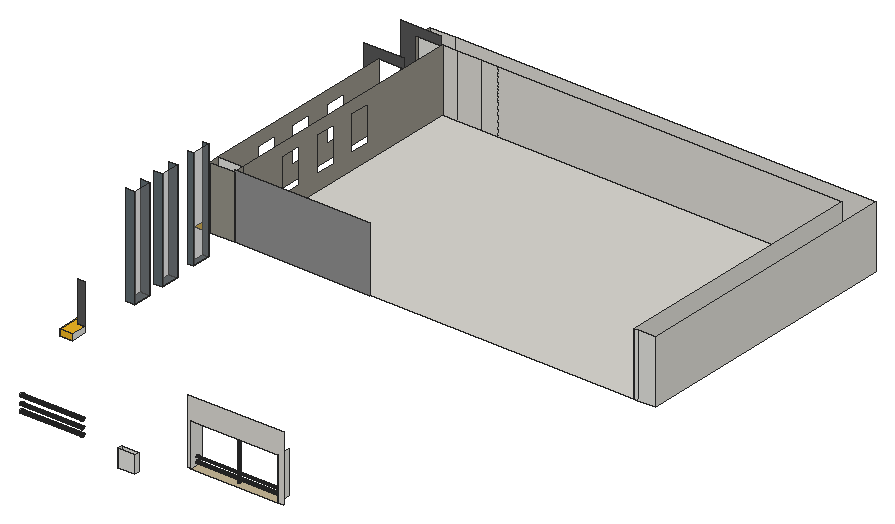
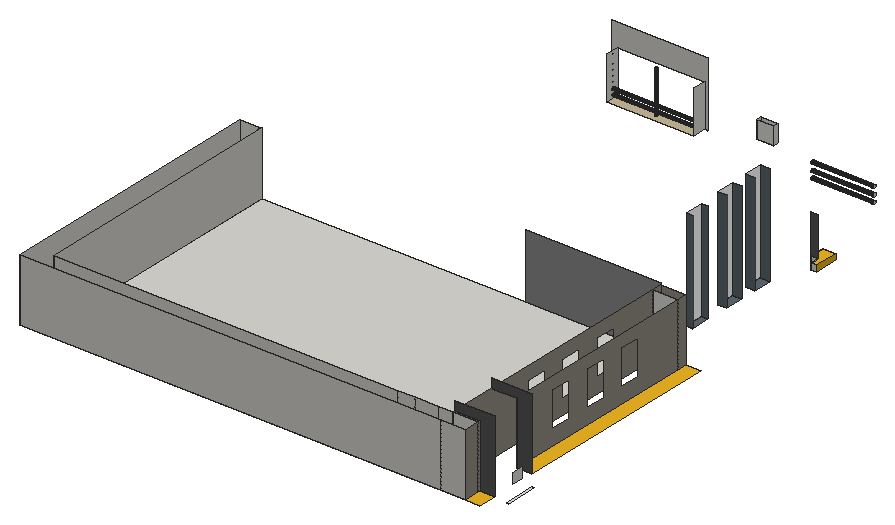
# SketchUp Ruby script. Lengths in inches.
U = 1.inch
M = Sketchup.active_model
def pt(a) = Geom::Point3d.new(a.map { |v| v * U })
def face(e, loops, mat)
  f = e.add_face(loops[0].map { |a| pt(a) })
  loops[1..].each { |l| e.add_face(l.map { |a| pt(a) }).erase! }
  f.material = f.back_material = mat if mat
  f
end
# faces: each face lists its corners as indices into pts; further lists are holes
def faces(e, pts, list, mat = nil) = list.each { |f| face(e, (f[0].is_a?(Array) ? f : [f]).map { |l| l.map { |i| pts[i] } }, mat) }
# xy, xz, yz: faces in a plane at the given z, y or x. An outline is a flat list of corners, or four numbers for a rectangle; further outlines are holes
def ring(l) = l.size == 4 ? [[l[0], l[1]], [l[2], l[1]], [l[2], l[3]], [l[0], l[3]]] : l.each_slice(2).to_a
def flat(e, list, mat, &to3) = list.each { |f| face(e, (f[0].is_a?(Array) ? f : [f]).map { |l| ring(l).map { |u, v| to3.(u, v) } }, mat) }
def xy(e, z, list, mat = nil) = flat(e, list, mat) { |x, y| [x, y, z] }
def xz(e, y, list, mat = nil) = flat(e, list, mat) { |x, z| [x, y, z] }
def yz(e, x, list, mat = nil) = flat(e, list, mat) { |y, z| [x, y, z] }
def lines(e, pts, list) = list.each { |a, b| e.add_line(pt(pts[a]), pt(pts[b])) }
# prism: a flat outline (further loops are holes) pulled along v
def prism(e, loops, v, mat = nil)
  f = face(e, loops, mat); d = Geom::Vector3d.new(v.map { |x| x * U })
  f.pushpull(f.normal.samedirection?(d) ? d.length : -d.length)
end
def box(e, o, s, mat = nil) = prism(e, [[o, [o[0] + s[0], o[1], o[2]], [o[0] + s[0], o[1] + s[1], o[2]], [o[0], o[1] + s[1], o[2]]]], [0, 0, s[2]], mat)
def at(x, y, z, deg = 0) = Geom::Transformation.translation(pt([x, y, z])) * Geom::Transformation.rotation(ORIGIN, Z_AXIS, deg.degrees)
def axes(o, x, y, z) = Geom::Transformation.new([*x, 0, *y, 0, *z, 0, *pt(o).to_a, 1])
def part(name) = M.definitions.add(name)
# library, detail: a bought-in or finely detailed component or shape, given as its bounding box
def library(name, o, s) = part(name).tap { |d| box(d.entities, o, s) }
def detail(e, o, s) = box(e.add_group.entities, o, s)
def put(e, d, t, mat = nil) = e.add_instance(d, t).tap { |i| i.material = mat if mat }
def group(e, t, mat = nil) = e.add_group.tap { |g| g.transformation = t; g.material = mat if mat }.entities
root = M.entities
M.materials.add("[0045_Goldenrod]").color = [239, 181, 35]
M.materials.add("[Color M04]").color = [142, 142, 142]
M.materials.add("[Color M06]").color = [86, 86, 86]
M.materials.add("[Color M07]").color = [58, 58, 58]
M.materials.add("[Formica Graystone]").color = [149, 146, 135]
M.materials.add("[Formica Speckled Grey]").color = [94, 105, 111]
M.materials.add("[Quartz Light Brown]").color = [199, 184, 152]
M.materials.add("[Terrazzo Tile Light]").color = [219, 217, 210]
M.materials.add("[Translucent Glass Gray]1").color = [128, 128, 128]
M.materials["[Translucent Glass Gray]1"].alpha = 0.5
xy(root,388.58,[[0,731.17,2.5625,767.73]])
xy(root,390.15,[[220.22,108.25,239.85,114.1875]])
xy(root,396.69,[[329.08,144.78,328.77,144.82,328.48,144.9375,328.24,145.125,328.05,145.37,327.93,145.66,327.89,145.96,327.93,146.27,328.05,146.56,328.24,146.8,328.48,146.99,328.77,147.11,329.08,147.15,329.38,147.11,329.67,146.99,329.91,146.8,330.1,146.56,330.22,146.27,330.26,145.96,330.22,145.66,330.1,145.37,329.91,145.125,329.67,144.9375,329.38,144.82]])
xy(root,396.69,[[[280.22,138.52,379.09,153.42],[329.08,144.78,328.77,144.82,328.48,144.9375,328.24,145.125,328.05,145.37,327.93,145.66,327.89,145.96,327.93,146.27,328.05,146.56,328.24,146.8,328.48,146.99,328.77,147.11,329.08,147.15,329.38,147.11,329.67,146.99,329.91,146.8,330.1,146.56,330.22,146.27,330.26,145.96,330.22,145.66,330.1,145.37,329.91,145.125,329.67,144.9375,329.38,144.82]]],"[Quartz Light Brown]")
xy(root,396.875,[[25.28,483.625,53.375,495.58],[509.21,483.625,509.21,779.875,25.28,779.875,25.28,797.6875,533.375,797.6875,533.375,483.625]])
xy(root,396.875,[[8.375,483.625,25.28,724.47],[8.375,777.2,25.28,797.6875]],"[0045_Goldenrod]")
xy(root,396.875,[[53.375,483.625,509.21,779.875]],"[Terrazzo Tile Light]")
xy(root,397.66,[[38.625,253.03,38.625,280.03,45.3125,280.03,45.3125,270.46,53.375,270.46,53.375,253.03]],"[0045_Goldenrod]")
xy(root,404.29,[[53.375,329.18,63.8125,350.43],[53.375,369.37,62.6875,390.62],[53.375,417,60.4375,438.25]],"[Formica Speckled Grey]")
xy(root,404.47,[[38.625,253.03,53.375,253.03,53.375,270.46,45.3125,270.46,45.3125,280.03,38.625,280.03]],"[0045_Goldenrod]")
xz(root,108.25,[[220.22,390.15,239.85,409.78]])
xz(root,114.1875,[[220.22,390.15,239.85,409.78]])
xz(root,138.52,[[276.16,396.69,280.22,396.69,280.22,445.19,379.09,445.19,379.09,396.69,385.17,396.69,385.17,471,276.16,471]],"[Terrazzo Tile Light]")
xz(root,253.03,[[38.625,397.66,53.375,404.47]],"[0045_Goldenrod]")
xz(root,270.46,[[45.3125,397.66,53.375,404.47]])
xz(root,270.46,[[45.3125,404.47,53.375,449.66]],"[Color M06]")
xz(root,280.03,[[38.625,397.66,45.3125,404.47]])
xz(root,329.18,[[53.375,404.29,63.8125,519.67]],"[Formica Speckled Grey]")
xz(root,350.43,[[53.375,404.29,63.8125,519.67]],"[Formica Speckled Grey]")
xz(root,369.37,[[53.375,404.29,62.6875,519.67]],"[Formica Speckled Grey]")
xz(root,390.62,[[53.375,404.29,62.6875,519.67]],"[Formica Speckled Grey]")
xz(root,417,[[53.375,404.29,60.4375,519.67]],"[Formica Speckled Grey]")
xz(root,438.25,[[53.375,404.29,60.4375,519.67]],"[Formica Speckled Grey]")
xz(root,483.625,[[509.21,396.875,513.45,468.5],[513.45,396.875,533.375,468.5]])
xz(root,483.625,[[53.375,396.875,208.03,471]],"[Color M04]")
xz(root,483.625,[[25.28,396.875,53.375,468.5]],"[Formica Graystone]")
xz(root,495.58,[[25.28,396.875,53.375,468.5]])
xz(root,724.47,[[8.375,396.875,25.28,396.875,25.28,468.5,53.375,468.5,53.375,479.1875,8.375,479.1875]],"[Color M06]")
xz(root,777.2,[[8.375,396.875,8.375,479.1875,53.375,479.1875,53.375,468.5,25.28,468.5,25.28,396.875]],"[Color M06]")
xz(root,779.875,[[25.28,396.875,53.375,468.5]])
xz(root,779.875,[[53.375,396.875,70.21,468.5],[70.21,396.875,97.02,468.5],[97.02,396.875,116.75,468.5],[116.75,396.875,509.21,468.5]],"[Terrazzo Tile Light]")
xz(root,797.6875,[[25.28,396.875,53.375,468.5],[53.375,396.875,533.375,468.5]],"[Terrazzo Tile Light]")
yz(root,2.5625,[[745.75,403.69,759.0625,415.44]])
yz(root,25.28,[[483.625,396.875,495.58,468.5],[[495.58,396.875,724.47,468.5],[649.81,414.79,673.99,454.59],[600.93,414.79,625.12,454.59],[551.74,414.79,575.93,454.59]],[777.2,396.875,779.875,468.5],[779.875,396.875,797.6875,468.5]],"[Formica Graystone]")
yz(root,38.625,[[253.03,397.66,280.03,404.47]],"[0045_Goldenrod]")
yz(root,45.3125,[[270.46,397.66,280.03,404.47]])
yz(root,53.375,[[253.03,397.66,270.46,404.47]])
yz(root,53.375,[[483.625,396.875,495.58,468.5],[[495.58,396.875,779.875,468.5],[649.81,414.79,673.99,454.59],[600.93,414.79,625.12,454.59],[551.74,414.79,575.93,454.59]]],"[Formica Graystone]")
yz(root,60.4375,[[417,404.29,438.25,519.67]],"[Translucent Glass Gray]1")
yz(root,62.6875,[[369.37,404.29,390.62,519.67]],"[Translucent Glass Gray]1")
yz(root,63.8125,[[329.18,404.29,350.43,519.67]],"[Translucent Glass Gray]1")
yz(root,87.31,[[136.99,387.18,136.55,387.24,136.14,387.41,135.79,387.67,135.52,388.02,135.36,388.43,135.3,388.87,135.36,389.3,135.52,389.71,135.79,390.06,136.14,390.33,136.55,390.5,136.99,390.55,137.42,390.5,137.83,390.33,138.18,390.06,138.45,389.71,138.62,389.3,138.67,388.87,138.62,388.43,138.45,388.02,138.18,387.67,137.83,387.41,137.42,387.24],[136.99,394.8,136.55,394.86,136.14,395.03,135.79,395.3,135.52,395.65,135.36,396.06,135.3,396.49,135.36,396.93,135.52,397.34,135.79,397.69,136.14,397.95,136.55,398.12,136.99,398.18,137.42,398.12,137.83,397.95,138.18,397.69,138.45,397.34,138.62,396.93,138.67,396.49,138.62,396.06,138.45,395.65,138.18,395.3,137.83,395.03,137.42,394.86],[136.99,403.55,136.55,403.61,136.14,403.78,135.79,404.05,135.52,404.4,135.36,404.81,135.3,405.24,135.36,405.68,135.52,406.09,135.79,406.44,136.14,406.7,136.55,406.87,136.99,406.93,137.42,406.87,137.83,406.7,138.18,406.44,138.45,406.09,138.62,405.68,138.67,405.24,138.62,404.81,138.45,404.4,138.18,404.05,137.83,403.78,137.42,403.61]])
yz(root,220.22,[[108.25,390.15,114.1875,409.78]])
yz(root,239.85,[[108.25,390.15,114.1875,409.78]])
yz(root,280.22,[[[138.52,396.69,153.42,445.19],[145.73,399.5,145.38,399.55,145.05,399.6875,144.76,399.91,144.54,400.19,144.41,400.52,144.36,400.88,144.41,401.23,144.54,401.57,144.76,401.85,145.05,402.07,145.38,402.21,145.73,402.25,146.09,402.21,146.42,402.07,146.71,401.85,146.92,401.57,147.0625,401.23,147.11,400.88,147.0625,400.52,146.92,400.19,146.71,399.91,146.42,399.6875,146.09,399.55],[145.73,434.63,145.38,434.67,145.05,434.8125,144.76,435.03,144.54,435.32,144.41,435.65,144.36,436,144.41,436.36,144.54,436.69,144.76,436.97,145.05,437.19,145.38,437.33,145.73,437.38,146.09,437.33,146.42,437.19,146.71,436.97,146.92,436.69,147.0625,436.36,147.11,436,147.0625,435.65,146.92,435.32,146.71,435.03,146.42,434.8125,146.09,434.67],[145.73,405.25,145.38,405.3,145.05,405.4375,144.76,405.66,144.54,405.94,144.41,406.27,144.36,406.63,144.41,406.98,144.54,407.32,144.76,407.6,145.05,407.82,145.38,407.96,145.73,408,146.09,407.96,146.42,407.82,146.71,407.6,146.92,407.32,147.0625,406.98,147.11,406.63,147.0625,406.27,146.92,405.94,146.71,405.66,146.42,405.4375,146.09,405.3],[145.73,429.69,145.38,429.74,145.05,429.875,144.76,430.09,144.54,430.38,144.41,430.71,144.36,431.07,144.41,431.42,144.54,431.75,144.76,432.04,145.05,432.26,145.38,432.39,145.73,432.44,146.09,432.39,146.42,432.26,146.71,432.04,146.92,431.75,147.0625,431.42,147.11,431.07,147.0625,430.71,146.92,430.38,146.71,430.09,146.42,429.875,146.09,429.74],[145.61,411.18,145.26,411.23,144.93,411.37,144.64,411.59,144.42,411.87,144.29,412.2,144.24,412.56,144.29,412.92,144.42,413.25,144.64,413.53,144.93,413.75,145.26,413.89,145.61,413.93,145.97,413.89,146.3,413.75,146.59,413.53,146.81,413.25,146.94,412.92,146.99,412.56,146.94,412.2,146.81,411.87,146.59,411.59,146.3,411.37,145.97,411.23],[145.61,424.12,145.26,424.17,144.93,424.31,144.64,424.52,144.42,424.81,144.29,425.14,144.24,425.5,144.29,425.85,144.42,426.18,144.64,426.47,144.93,426.6875,145.26,426.83,145.61,426.87,145.97,426.83,146.3,426.6875,146.59,426.47,146.81,426.18,146.94,425.85,146.99,425.5,146.94,425.14,146.81,424.81,146.59,424.52,146.3,424.31,145.97,424.17],[145.61,417.75,145.26,417.79,144.93,417.93,144.64,418.15,144.42,418.43,144.29,418.77,144.24,419.12,144.29,419.48,144.42,419.81,144.64,420.09,144.93,420.3125,145.26,420.45,145.61,420.5,145.97,420.45,146.3,420.3125,146.59,420.09,146.81,419.81,146.94,419.48,146.99,419.12,146.94,418.77,146.81,418.43,146.59,418.15,146.3,417.93,145.97,417.79],[145.73,439.94,145.38,439.99,145.05,440.125,144.76,440.34,144.54,440.63,144.41,440.96,144.36,441.32,144.41,441.67,144.54,442,144.76,442.29,145.05,442.51,145.38,442.64,145.73,442.69,146.09,442.64,146.42,442.51,146.71,442.29,146.92,442,147.0625,441.67,147.11,441.32,147.0625,440.96,146.92,440.63,146.71,440.34,146.42,440.125,146.09,439.99]],[145.73,399.5,145.38,399.55,145.05,399.6875,144.76,399.91,144.54,400.19,144.41,400.52,144.36,400.88,144.41,401.23,144.54,401.57,144.76,401.85,145.05,402.07,145.38,402.21,145.73,402.25,146.09,402.21,146.42,402.07,146.71,401.85,146.92,401.57,147.0625,401.23,147.11,400.88,147.0625,400.52,146.92,400.19,146.71,399.91,146.42,399.6875,146.09,399.55],[145.73,405.25,145.38,405.3,145.05,405.4375,144.76,405.66,144.54,405.94,144.41,406.27,144.36,406.63,144.41,406.98,144.54,407.32,144.76,407.6,145.05,407.82,145.38,407.96,145.73,408,146.09,407.96,146.42,407.82,146.71,407.6,146.92,407.32,147.0625,406.98,147.11,406.63,147.0625,406.27,146.92,405.94,146.71,405.66,146.42,405.4375,146.09,405.3]])
yz(root,379.09,[[[138.52,396.69,153.42,445.19],[145.73,439.94,146.09,439.99,146.42,440.125,146.71,440.34,146.92,440.63,147.0625,440.96,147.11,441.32,147.0625,441.67,146.92,442,146.71,442.29,146.42,442.51,146.09,442.64,145.73,442.69,145.38,442.64,145.05,442.51,144.76,442.29,144.54,442,144.41,441.67,144.36,441.32,144.41,440.96,144.54,440.63,144.76,440.34,145.05,440.125,145.38,439.99],[145.73,434.63,146.09,434.67,146.42,434.8125,146.71,435.03,146.92,435.32,147.0625,435.65,147.11,436,147.0625,436.36,146.92,436.69,146.71,436.97,146.42,437.19,146.09,437.33,145.73,437.38,145.38,437.33,145.05,437.19,144.76,436.97,144.54,436.69,144.41,436.36,144.36,436,144.41,435.65,144.54,435.32,144.76,435.03,145.05,434.8125,145.38,434.67],[145.73,429.69,146.09,429.74,146.42,429.875,146.71,430.09,146.92,430.38,147.0625,430.71,147.11,431.07,147.0625,431.42,146.92,431.75,146.71,432.04,146.42,432.26,146.09,432.39,145.73,432.44,145.38,432.39,145.05,432.26,144.76,432.04,144.54,431.75,144.41,431.42,144.36,431.07,144.41,430.71,144.54,430.38,144.76,430.09,145.05,429.875,145.38,429.74],[145.61,424.12,145.97,424.17,146.3,424.31,146.59,424.52,146.81,424.81,146.94,425.14,146.99,425.5,146.94,425.85,146.81,426.18,146.59,426.47,146.3,426.6875,145.97,426.83,145.61,426.87,145.26,426.83,144.93,426.6875,144.64,426.47,144.42,426.18,144.29,425.85,144.24,425.5,144.29,425.14,144.42,424.81,144.64,424.52,144.93,424.31,145.26,424.17],[145.61,417.75,145.97,417.79,146.3,417.93,146.59,418.15,146.81,418.43,146.94,418.77,146.99,419.12,146.94,419.48,146.81,419.81,146.59,420.09,146.3,420.3125,145.97,420.45,145.61,420.5,145.26,420.45,144.93,420.3125,144.64,420.09,144.42,419.81,144.29,419.48,144.24,419.12,144.29,418.77,144.42,418.43,144.64,418.15,144.93,417.93,145.26,417.79],[145.61,411.18,145.97,411.23,146.3,411.37,146.59,411.59,146.81,411.87,146.94,412.2,146.99,412.56,146.94,412.92,146.81,413.25,146.59,413.53,146.3,413.75,145.97,413.89,145.61,413.93,145.26,413.89,144.93,413.75,144.64,413.53,144.42,413.25,144.29,412.92,144.24,412.56,144.29,412.2,144.42,411.87,144.64,411.59,144.93,411.37,145.26,411.23],[145.73,405.25,146.09,405.3,146.42,405.4375,146.71,405.66,146.92,405.94,147.0625,406.27,147.11,406.63,147.0625,406.98,146.92,407.32,146.71,407.6,146.42,407.82,146.09,407.96,145.73,408,145.38,407.96,145.05,407.82,144.76,407.6,144.54,407.32,144.41,406.98,144.36,406.63,144.41,406.27,144.54,405.94,144.76,405.66,145.05,405.4375,145.38,405.3],[145.73,399.5,146.09,399.55,146.42,399.6875,146.71,399.91,146.92,400.19,147.0625,400.52,147.11,400.88,147.0625,401.23,146.92,401.57,146.71,401.85,146.42,402.07,146.09,402.21,145.73,402.25,145.38,402.21,145.05,402.07,144.76,401.85,144.54,401.57,144.41,401.23,144.36,400.88,144.41,400.52,144.54,400.19,144.76,399.91,145.05,399.6875,145.38,399.55]]])
yz(root,509.21,[[483.625,396.875,779.875,468.5]],"[Terrazzo Tile Light]")
yz(root,533.375,[[483.625,396.875,797.6875,468.5]],"[Terrazzo Tile Light]")
p = [[87.31,136.14,387.41],[87.31,136.55,387.24],[158.23,136.55,387.24],[158.23,136.14,387.41],[87.31,136.99,387.18],[158.23,136.99,387.18],
  [87.31,137.42,387.24],[158.23,137.42,387.24],[87.31,137.83,387.41],[158.23,137.83,387.41],[87.31,135.79,387.67],[158.23,135.79,387.67],
  [87.31,138.18,387.67],[158.23,138.18,387.67],[87.31,135.52,388.02],[158.23,135.52,388.02],[87.31,138.45,388.02],[158.23,138.45,388.02],
  [87.31,135.36,388.43],[158.23,135.36,388.43],[87.31,138.62,388.43],[158.23,138.62,388.43],[87.31,135.3,388.87],[158.23,135.3,388.87],
  [87.31,138.67,388.87],[158.23,138.67,388.87],[87.31,135.36,389.3],[158.23,135.36,389.3],[87.31,138.62,389.3],[158.23,138.62,389.3],
  [87.31,135.52,389.71],[158.23,135.52,389.71],[87.31,138.45,389.71],[158.23,138.45,389.71],[87.31,135.79,390.06],[158.23,135.79,390.06],
  [87.31,138.18,390.06],[158.23,138.18,390.06],[87.31,136.14,390.33],[158.23,136.14,390.33],[87.31,137.83,390.33],[158.23,137.83,390.33],
  [87.31,136.55,390.5],[158.23,136.55,390.5],[87.31,137.42,390.5],[158.23,137.42,390.5],[87.31,136.99,390.55],[158.23,136.99,390.55],
  [87.31,136.55,394.86],[87.31,136.99,394.8],[158.23,136.99,394.8],[158.23,136.55,394.86],[87.31,137.42,394.86],[158.23,137.42,394.86],
  [87.31,136.14,395.03],[158.23,136.14,395.03],[87.31,137.83,395.03],[158.23,137.83,395.03],[87.31,135.79,395.3],[158.23,135.79,395.3],
  [87.31,138.18,395.3],[158.23,138.18,395.3],[87.31,135.52,395.65],[158.23,135.52,395.65],[87.31,138.45,395.65],[158.23,138.45,395.65],
  [87.31,135.36,396.06],[158.23,135.36,396.06],[87.31,138.62,396.06],[158.23,138.62,396.06],[87.31,135.3,396.49],[158.23,135.3,396.49],
  [87.31,138.67,396.49],[158.23,138.67,396.49],[87.31,135.36,396.93],[158.23,135.36,396.93],[87.31,138.62,396.93],[158.23,138.62,396.93],
  [328.48,144.9375,396.69],[328.77,144.82,396.69],[328.77,144.82,445.19],[328.48,144.9375,445.19],[329.08,144.78,396.69],[329.08,144.78,445.19],
  [329.38,144.82,396.69],[329.38,144.82,445.19],[329.67,144.9375,396.69],[329.67,144.9375,445.19],[328.24,145.125,396.69],[328.24,145.125,445.19],
  [329.91,145.125,396.69],[329.91,145.125,445.19],[328.05,145.37,396.69],[328.05,145.37,445.19],[330.1,145.37,396.69],[330.1,145.37,445.19],
  [327.93,145.66,396.69],[327.93,145.66,445.19],[330.22,145.66,396.69],[330.22,145.66,445.19],[327.89,145.96,396.69],[327.89,145.96,445.19],
  [330.26,145.96,396.69],[330.26,145.96,445.19],[327.93,146.27,396.69],[327.93,146.27,445.19],[330.22,146.27,396.69],[330.22,146.27,445.19],
  [328.05,146.56,396.69],[328.05,146.56,445.19],[330.1,146.56,396.69],[330.1,146.56,445.19],[328.24,146.8,396.69],[328.24,146.8,445.19],
  [329.91,146.8,396.69],[329.91,146.8,445.19],[328.48,146.99,396.69],[328.48,146.99,445.19],[329.67,146.99,396.69],[329.67,146.99,445.19],
  [328.77,147.11,396.69],[328.77,147.11,445.19],[329.38,147.11,396.69],[329.38,147.11,445.19],[329.08,147.15,396.69],[329.08,147.15,445.19],
  [87.31,135.52,397.34],[158.23,135.52,397.34],[87.31,138.45,397.34],[158.23,138.45,397.34],[87.31,135.79,397.69],[158.23,135.79,397.69],
  [87.31,138.18,397.69],[158.23,138.18,397.69],[87.31,136.14,397.95],[158.23,136.14,397.95],[87.31,137.83,397.95],[158.23,137.83,397.95],
  [87.31,136.55,398.12],[158.23,136.55,398.12],[87.31,137.42,398.12],[158.23,137.42,398.12],[87.31,136.99,398.18],[158.23,136.99,398.18],
  [280.22,145.05,399.6875],[280.22,145.38,399.55],[379.09,145.38,399.55],[379.09,145.05,399.6875],[280.22,145.73,399.5],[379.09,145.73,399.5],
  [280.22,146.09,399.55],[379.09,146.09,399.55],[280.22,146.42,399.6875],[379.09,146.42,399.6875],[280.22,144.76,399.91],[379.09,144.76,399.91],
  [280.22,146.71,399.91],[379.09,146.71,399.91],[280.22,144.54,400.19],[379.09,144.54,400.19],[280.22,146.92,400.19],[379.09,146.92,400.19],
  [280.22,144.41,400.52],[379.09,144.41,400.52],[280.22,147.0625,400.52],[379.09,147.0625,400.52],[280.22,144.36,400.88],[379.09,144.36,400.88],
  [280.22,147.11,400.88],[379.09,147.11,400.88],[280.22,144.41,401.23],[379.09,144.41,401.23],[280.22,147.0625,401.23],[379.09,147.0625,401.23],
  [280.22,144.54,401.57],[379.09,144.54,401.57],[280.22,146.92,401.57],[379.09,146.92,401.57],[280.22,144.76,401.85],[379.09,144.76,401.85],
  [280.22,146.71,401.85],[379.09,146.71,401.85],[280.22,145.05,402.07],[379.09,145.05,402.07],[280.22,146.42,402.07],[379.09,146.42,402.07],
  [280.22,145.38,402.21],[379.09,145.38,402.21],[280.22,146.09,402.21],[379.09,146.09,402.21],[280.22,145.73,402.25],[379.09,145.73,402.25],
  [87.31,136.14,403.78],[87.31,136.55,403.61],[158.23,136.55,403.61],[158.23,136.14,403.78],[87.31,136.99,403.55],[158.23,136.99,403.55],
  [87.31,137.42,403.61],[158.23,137.42,403.61],[87.31,137.83,403.78],[158.23,137.83,403.78],[87.31,135.79,404.05],[158.23,135.79,404.05],
  [87.31,138.18,404.05],[158.23,138.18,404.05],[87.31,135.52,404.4],[158.23,135.52,404.4],[87.31,138.45,404.4],[158.23,138.45,404.4],
  [87.31,135.36,404.81],[158.23,135.36,404.81],[87.31,138.62,404.81],[158.23,138.62,404.81],[87.31,135.3,405.24],[158.23,135.3,405.24],
  [87.31,138.67,405.24],[158.23,138.67,405.24],[87.31,135.36,405.68],[158.23,135.36,405.68],[87.31,138.62,405.68],[158.23,138.62,405.68],
  [280.22,145.05,405.4375],[280.22,145.38,405.3],[379.09,145.38,405.3],[379.09,145.05,405.4375],[280.22,145.73,405.25],[379.09,145.73,405.25],
  [280.22,146.09,405.3],[379.09,146.09,405.3],[280.22,146.42,405.4375],[379.09,146.42,405.4375],[280.22,144.76,405.66],[379.09,144.76,405.66],
  [280.22,146.71,405.66],[379.09,146.71,405.66],[87.31,135.52,406.09],[158.23,135.52,406.09],[87.31,138.45,406.09],[158.23,138.45,406.09],
  [280.22,144.54,405.94],[379.09,144.54,405.94],[280.22,146.92,405.94],[379.09,146.92,405.94],[280.22,144.41,406.27],[379.09,144.41,406.27],
  [280.22,147.0625,406.27],[379.09,147.0625,406.27],[87.31,135.79,406.44],[158.23,135.79,406.44],[87.31,138.18,406.44],[158.23,138.18,406.44],
  [280.22,144.36,406.63],[379.09,144.36,406.63],[280.22,147.11,406.63],[379.09,147.11,406.63],[87.31,136.14,406.7],[158.23,136.14,406.7],
  [87.31,137.83,406.7],[158.23,137.83,406.7],[280.22,144.41,406.98],[379.09,144.41,406.98],[280.22,147.0625,406.98],[379.09,147.0625,406.98],
  [87.31,136.55,406.87],[158.23,136.55,406.87],[87.31,137.42,406.87],[158.23,137.42,406.87],[87.31,136.99,406.93],[158.23,136.99,406.93],
  [280.22,144.54,407.32],[379.09,144.54,407.32],[280.22,146.92,407.32],[379.09,146.92,407.32],[280.22,144.76,407.6],[379.09,144.76,407.6],
  [280.22,146.71,407.6],[379.09,146.71,407.6],[280.22,145.05,407.82],[379.09,145.05,407.82],[280.22,146.42,407.82],[379.09,146.42,407.82],
  [280.22,145.38,407.96],[379.09,145.38,407.96],[280.22,146.09,407.96],[379.09,146.09,407.96],[280.22,145.73,408],[379.09,145.73,408]]
faces(root,p,[[0,1,2,3],[1,4,5,2],[4,6,7,5],[6,8,9,7],[10,0,3,11],[8,12,13,9],[14,10,11,15],[12,16,17,13],
  [18,14,15,19],[16,20,21,17],[22,18,19,23],[20,24,25,21],[26,22,23,27],[24,28,29,25],[30,26,27,31],[28,32,33,29],
  [34,30,31,35],[32,36,37,33],[38,34,35,39],[36,40,41,37],[42,38,39,43],[40,44,45,41],[46,42,43,47],[44,46,47,45],
  [48,49,50,51],[49,52,53,50],[54,48,51,55],[52,56,57,53],[58,54,55,59],[56,60,61,57],[62,58,59,63],[60,64,65,61],
  [66,62,63,67],[64,68,69,65],[70,66,67,71],[68,72,73,69],[74,70,71,75],[72,76,77,73],[78,79,80,81],[79,82,83,80],
  [82,84,85,83],[84,86,87,85],[88,78,81,89],[86,90,91,87],[92,88,89,93],[90,94,95,91],[96,92,93,97],[94,98,99,95],
  [100,96,97,101],[98,102,103,99],[104,100,101,105],[102,106,107,103],[108,104,105,109],[106,110,111,107],[112,108,109,113],[110,114,115,111],
  [116,112,113,117],[114,118,119,115],[120,116,117,121],[118,122,123,119],[124,120,121,125],[122,124,125,123],[126,74,75,127],[76,128,129,77],
  [130,126,127,131],[128,132,133,129],[134,130,131,135],[132,136,137,133],[138,134,135,139],[136,140,141,137],[142,138,139,143],[140,142,143,141],
  [144,145,146,147],[145,148,149,146],[148,150,151,149],[150,152,153,151],[154,144,147,155],[152,156,157,153],[158,154,155,159],[156,160,161,157],
  [162,158,159,163],[160,164,165,161],[166,162,163,167],[164,168,169,165],[170,166,167,171],[168,172,173,169],[174,170,171,175],[172,176,177,173],
  [178,174,175,179],[176,180,181,177],[182,178,179,183],[180,184,185,181],[186,182,183,187],[184,188,189,185],[190,186,187,191],[188,190,191,189],
  [192,193,194,195],[193,196,197,194],[196,198,199,197],[198,200,201,199],[202,192,195,203],[200,204,205,201],[206,202,203,207],[204,208,209,205],
  [210,206,207,211],[208,212,213,209],[214,210,211,215],[212,216,217,213],[218,214,215,219],[216,220,221,217],[222,223,224,225],[223,226,227,224],
  [226,228,229,227],[228,230,231,229],[232,222,225,233],[230,234,235,231],[236,218,219,237],[220,238,239,221],[240,232,233,241],[234,242,243,235],
  [244,240,241,245],[242,246,247,243],[248,236,237,249],[238,250,251,239],[252,244,245,253],[246,254,255,247],[256,248,249,257],[250,258,259,251],
  [260,252,253,261],[254,262,263,255],[264,256,257,265],[258,266,267,259],[268,264,265,269],[266,268,269,267],[270,260,261,271],[262,272,273,263],
  [274,270,271,275],[272,276,277,273],[278,274,275,279],[276,280,281,277],[282,278,279,283],[280,284,285,281],[286,282,283,287],[284,286,287,285]],"[Color M07]")
